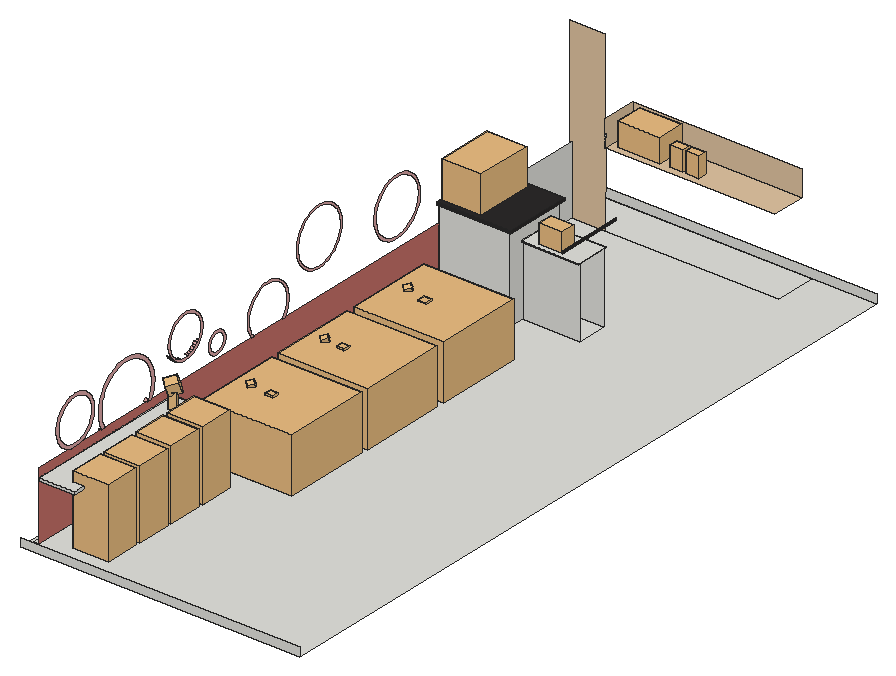
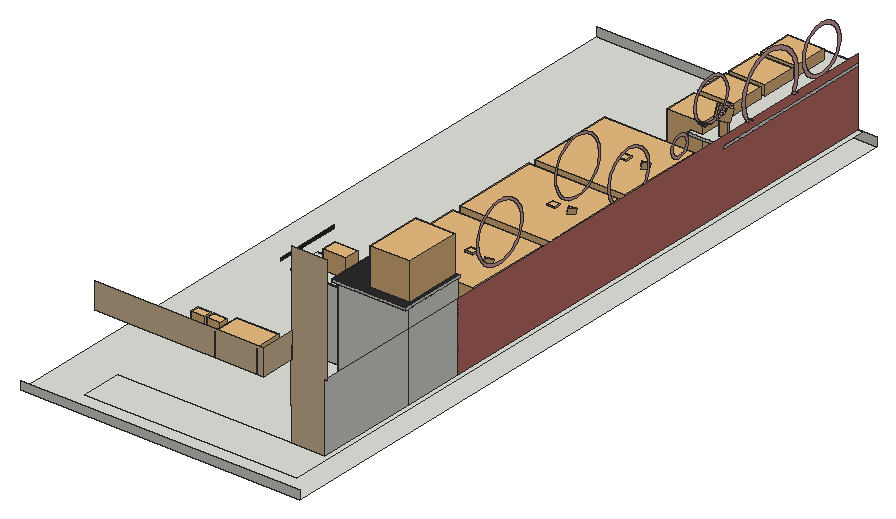
# SketchUp Ruby script. Lengths in inches.
U = 1.inch
M = Sketchup.active_model
def pt(a) = Geom::Point3d.new(a.map { |v| v * U })
def face(e, loops, mat)
  f = e.add_face(loops[0].map { |a| pt(a) })
  loops[1..].each { |l| e.add_face(l.map { |a| pt(a) }).erase! }
  f.material = f.back_material = mat if mat
  f
end
# faces: each face lists its corners as indices into pts; further lists are holes
def faces(e, pts, list, mat = nil) = list.each { |f| face(e, (f[0].is_a?(Array) ? f : [f]).map { |l| l.map { |i| pts[i] } }, mat) }
# xy, xz, yz: faces in a plane at the given z, y or x. An outline is a flat list of corners, or four numbers for a rectangle; further outlines are holes
def ring(l) = l.size == 4 ? [[l[0], l[1]], [l[2], l[1]], [l[2], l[3]], [l[0], l[3]]] : l.each_slice(2).to_a
def flat(e, list, mat, &to3) = list.each { |f| face(e, (f[0].is_a?(Array) ? f : [f]).map { |l| ring(l).map { |u, v| to3.(u, v) } }, mat) }
def xy(e, z, list, mat = nil) = flat(e, list, mat) { |x, y| [x, y, z] }
def xz(e, y, list, mat = nil) = flat(e, list, mat) { |x, z| [x, y, z] }
def yz(e, x, list, mat = nil) = flat(e, list, mat) { |y, z| [x, y, z] }
def lines(e, pts, list) = list.each { |a, b| e.add_line(pt(pts[a]), pt(pts[b])) }
# prism: a flat outline (further loops are holes) pulled along v
def prism(e, loops, v, mat = nil)
  f = face(e, loops, mat); d = Geom::Vector3d.new(v.map { |x| x * U })
  f.pushpull(f.normal.samedirection?(d) ? d.length : -d.length)
end
def box(e, o, s, mat = nil) = prism(e, [[o, [o[0] + s[0], o[1], o[2]], [o[0] + s[0], o[1] + s[1], o[2]], [o[0], o[1] + s[1], o[2]]]], [0, 0, s[2]], mat)
def at(x, y, z, deg = 0) = Geom::Transformation.translation(pt([x, y, z])) * Geom::Transformation.rotation(ORIGIN, Z_AXIS, deg.degrees)
def axes(o, x, y, z) = Geom::Transformation.new([*x, 0, *y, 0, *z, 0, *pt(o).to_a, 1])
def part(name) = M.definitions.add(name)
# library, detail: a bought-in or finely detailed component or shape, given as its bounding box
def library(name, o, s) = part(name).tap { |d| box(d.entities, o, s) }
def detail(e, o, s) = box(e.add_group.entities, o, s)
def put(e, d, t, mat = nil) = e.add_instance(d, t).tap { |i| i.material = mat if mat }
def group(e, t, mat = nil) = e.add_group.tap { |g| g.transformation = t; g.material = mat if mat }.entities
root = M.entities
M.materials.add("Generic").color = [224, 169, 169]
M.materials.add("Generic\#1").color = [44, 42, 42]
M.materials.add("Generic\#3").color = [224, 196, 161]
M.materials.add("Material__1").color = [51, 42, 44]
M.materials.add("Material__2").color = [97, 132, 37]
M.materials.add("[Wood Floor Dark]").color = [198, 114, 106]
c1 = library("\#1",[-138.85,-135.75,0],[277.7,270.97,9.64])
c2 = library("\#2",[-34.84,-73.35,-33.91],[69.68,146.26,68.31])
c3 = library("\#5",[-4127.85,-1300.75,-2324.72],[5349.84,4521.24,5423.31])
c4 = part("\#3")
put(c4.entities,c3,at(450.18,-1111.4375,0),"Material__2")
c5 = part("12")
put(c5.entities,c1,axes([-49.79,-36.9375,349.64],[0.59279,0,0],[0,0.59279,0],[0,0,0.59279]),"Material__1")
put(c5.entities,c2,axes([-39.24,-18.18,177.19],[1.20819,-2.09264,0],[0,0,2.41638],[2.09264,1.20819,0]))
put(c5.entities,c4,axes([-83.44,-46.04,442.44],[-0.03636,-0.03293,-0.01473],[-0.00083,-0.02391,0.05549],[0.02997,-0.02791,-0.01158]))
c6 = library("Group\#636",[0,0,0],[15.67,22.625,14.53])
c7 = library("Group\#669",[0,0,0],[8.6,8.6,4.41])
c8 = library("Group",[-8.82,-17.72,0],[17.64,35.44,18.29])
c9 = library("Tissue box",[0,0,0],[4.59,4,6.84])
c10 = library("Group\#25",[0,0,0],[61.25,59.29,37.22])
c11 = library("Group\#26",[0,0,0],[61.25,59.29,37.22])
c12 = library("Group\#23",[0,0,0],[61.25,59.29,37.22])
c13 = library("Espresso+machine+low+poly",[-3.8125,0,0],[25.21,40.375,21.95])
c14 = library("Group\#670",[0,0,0],[21.93,14.72,17.62])
c15 = library("Countertop blender",[-3.14,-3.14,0],[6.83,6.28,15])
xy(root,-6,[[0,0,190,490.125]])
xy(root,0,[[9,0.4375,12.375,0.4375,12.375,453.375,153.2,453.375,153.2,481.125,9,481.125],[60.5625,351.3,99.75,371.55]])
xy(root,38.39,[[12.375,0.4375,36.5,114.5]])
xy(root,40.64,[[12.375,0.4375,36.5,114.5]])
xy(root,46.5,[[12.375,27.54,12.625,34.125],[12.375,53.23,12.9375,56.0625],[12.375,91.96,12.9375,94.93]])
xy(root,47.6875,[[60.5625,350.05,99.75,351.3],[60.5625,351.3,99.75,371.55],[60.5625,371.55,99.75,372.8]])
xy(root,48.3125,[[60.5625,350.05,99.75,372.8]])
xy(root,50.68,[[35.21,453.375,150.42,476.6875]],"Generic\#3")
xy(root,58.4375,[[12.375,338.55,62.5625,340.55],[12.375,340.55,60.5625,382.3],[60.5625,340.55,62.5625,384.3],[12.375,382.3,60.5625,384.3]])
xy(root,60.3125,[[12.375,338.55,62.5625,384.3]],"Generic\#1")
xz(root,0,[[0,-6,190,0]])
xz(root,0.4375,[[12.375,38.39,36.5,40.64]])
xz(root,114.5,[[12.375,38.39,36.5,40.64]])
xz(root,338.55,[[12.375,58.4375,62.5625,60.3125]],"Generic\#1")
xz(root,340.55,[[12.375,0,60.5625,58.4375]])
xz(root,350.05,[[60.5625,47.6875,99.75,48.3125]])
xz(root,351.3,[[60.5625,0,99.75,47.6875]])
xz(root,371.55,[[60.5625,0,99.75,47.6875]])
xz(root,372.8,[[60.5625,47.6875,99.75,48.3125]])
xz(root,382.3,[[12.375,0,60.5625,58.4375]])
xz(root,384.3,[[12.375,58.4375,62.5625,60.3125]])
xz(root,453.375,[[34.92,50.68,35.21,50.68,34.93,68.36,34.92,68.36]])
xz(root,453.375,[[12.375,0,34.875,0,35.29,46.12,35.21,50.68,34.92,50.68,34.92,68.36,34.93,68.36,34.875,71.49,34.875,120,10.6875,120,10.6875,46.5,12.375,46.5]],"Generic\#3")
xz(root,476.6875,[[35.21,50.68,150.42,50.68,150.42,68.36,34.93,68.36]],"Generic\#3")
xz(root,490.125,[[0,-6,190,0]])
yz(root,12,[[[305.99,52.23,308.22,52.44,310.42,52.9,312.54,53.61,314.58,54.5625,316.49,55.74,318.25,57.12,319.85,58.7,321.26,60.44,322.45,62.34,323.43,64.36,324.17,66.48,324.66,68.67,324.89,70.9,324.875,73.14,324.6,75.37,324.08,77.55,323.31,79.66,322.3,81.66,321.07,83.54,319.64,85.27,318.02,86.82,316.23,88.17,314.3,89.31,312.25,90.23,310.11,90.91,307.91,91.33,305.68,91.51,303.43,91.43,301.22,91.09,299.05,90.5,296.97,89.67,294.99,88.61,293.15,87.33,291.47,85.85,289.96,84.18,288.66,82.36,287.57,80.39,286.71,78.32,286.1,76.16,285.73,73.95,285.625,71.71,285.77,69.47,286.17,67.26,286.82,65.12,287.71,63.06,288.83,61.11,290.16,59.31,291.69,57.67,293.4,56.21,295.26,54.96,297.25,53.93,299.35,53.13,301.52,52.58,303.74,52.28],[305.93,53.75,303.86,53.8,301.8125,54.07,299.81,54.58,297.87,55.32,296.03,56.27,294.32,57.43,292.74,58.77,291.33,60.28,290.1,61.95,289.07,63.74,288.25,65.64,287.65,67.62,287.28,69.66,287.15,71.72,287.25,73.79,287.58,75.83,288.15,77.82,288.94,79.73,289.95,81.54,291.15,83.23,292.54,84.76,294.09,86.13,295.79,87.3125,297.61,88.29,299.53,89.06,301.53,89.6,303.58,89.91,305.64,89.99,307.71,89.83,309.74,89.43,311.71,88.81,313.6,87.96,315.38,86.91,317.03,85.66,318.53,84.23,319.85,82.64,320.98,80.9,321.91,79.05,322.62,77.11,323.11,75.1,323.36,73.04,323.375,70.97,323.15,68.92,322.7,66.9,322.02,64.94,321.12,63.08,320.02,61.33,318.72,59.72,317.25,58.26,315.62,56.99,313.86,55.9,311.98,55.03,310.02,54.375,307.99,53.95]]],"Generic")
yz(root,12.1875,[[[239.61,63.57,241.81,63.77,243.97,64.23,246.06,64.93,248.0625,65.86,249.94,67.02,251.68,68.38,253.25,69.93,254.64,71.65,255.82,73.52,256.77,75.51,257.5,77.59,257.98,79.75,258.22,81.94,258.2,84.15,257.93,86.34,257.41,88.49,256.66,90.5625,255.67,92.54,254.46,94.39,253.05,96.08,251.45,97.61,249.69,98.95,247.79,100.07,245.78,100.97,243.67,101.64,241.5,102.06,239.3,102.23,237.09,102.15,234.91,101.82,232.78,101.24,230.73,100.42,228.78,99.38,226.97,98.12,225.3125,96.66,223.83,95.02,222.55,93.22,221.48,91.29,220.64,89.25,220.03,87.125,219.67,84.95,219.5625,82.74,219.71,80.54,220.1,78.37,220.74,76.25,221.61,74.22,222.71,72.3125,224.03,70.53,225.53,68.92,227.21,67.49,229.05,66.25,231.01,65.24,233.07,64.45,235.21,63.91,237.4,63.61],[239.5625,64.78,237.49,64.82,235.44,65.1,233.4375,65.61,231.5,66.35,229.66,67.3,227.95,68.45,226.37,69.8,224.96,71.3125,223.73,72.98,222.7,74.77,221.88,76.67,221.28,78.65,220.91,80.6875,220.78,82.75,220.88,84.82,221.22,86.86,221.78,88.85,222.57,90.76,223.58,92.57,224.78,94.26,226.17,95.79,227.72,97.16,229.42,98.34,231.24,99.32,233.16,100.09,235.16,100.63,237.21,100.94,239.28,101.02,241.34,100.86,243.37,100.46,245.34,99.84,247.23,98.99,249.01,97.9375,250.66,96.6875,252.16,95.26,253.48,93.66,254.61,91.93,255.54,90.08,256.25,88.14,256.74,86.13,256.99,84.07,257,82,256.78,79.95,256.33,77.93,255.65,75.97,254.75,74.11,253.65,72.36,252.35,70.75,250.88,69.29,249.25,68.01,247.49,66.93,245.61,66.06,243.65,65.4,241.62,64.98]]],"Generic")
yz(root,12.375,[[340.55,0,382.3,46.5],[382.3,0,453.375,46.5],[0.4375,38.39,114.5,40.64],[340.55,46.5,382.3,58.4375],[338.55,58.4375,384.3,60.3125]])
yz(root,12.375,[[181.21,46.5,182.81,46.5,181.875,47.65,180.875,49.23,180.06,50.9,179.45,52.66,179.04,54.48,178.84,56.33,178.85,58.19,179.07,60.04,179.5,61.85,180.14,63.6,180.97,65.27,181.98,66.83,183.17,68.27,184.52,69.56,186,70.69,187.6,71.64,189.3,72.4,191.07,72.97,192.9,73.33,194.75,73.48,196.62,73.41,198.46,73.14,200.26,72.65,201.99,71.97,203.63,71.09,205.16,70.03,206.5625,68.8,207.8125,67.42,208.9,65.91,209.81,64.28,210.52,62.5625,211.04,60.77,211.34,58.93,211.4375,57.07,211.32,55.22,210.99,53.38,210.46,51.6,209.72,49.89,208.8,48.27,207.7,46.77,207.45,46.5,209.04,46.5,209.84,47.59,210.84,49.33,211.63,51.17,212.21,53.09,212.56,55.07,212.6875,57.07,212.58,59.07,212.25,61.05,211.7,62.97,210.93,64.82,209.95,66.58,208.78,68.2,207.4375,69.69,205.93,71.01,204.28,72.15,202.51,73.1,200.65,73.84,198.71,74.36,196.73,74.65,194.73,74.72,192.73,74.5625,190.76,74.18,188.85,73.57,187.02,72.74,185.3,71.72,183.7,70.5,182.26,69.11,180.98,67.57,179.89,65.89,178.99,64.1,178.31,62.21,177.84,60.26,177.6,58.27,177.59,56.27,177.81,54.27,178.25,52.32,178.91,50.42,179.79,48.62,180.86,46.93],[[152.02,49.25,152.83,49.33,153.61,49.5,154.38,49.76,155.11,50.09,155.8,50.51,156.44,51,157.02,51.55,157.54,52.17,157.99,52.84,158.36,53.56,158.65,54.31,158.85,55.09,158.97,55.88,159,56.6875,158.94,57.49,158.79,58.28,158.56,59.06,158.24,59.8,157.85,60.5,157.375,61.15,156.84,61.75,156.23,62.28,155.58,62.75,154.87,63.14,154.13,63.45,153.35,63.67,152.5625,63.81,151.76,63.87,150.95,63.83,150.16,63.7,149.38,63.49,148.63,63.2,147.92,62.82,147.25,62.37,146.64,61.84,146.09,61.26,145.61,60.61,145.2,59.92,144.87,59.18,144.62,58.42,144.46,57.625,144.38,56.82,144.4,56.02,144.5,55.22,144.69,54.4375,144.97,53.68,145.32,52.96,145.76,52.28,146.26,51.65,146.84,51.09,147.47,50.59,148.15,50.16,148.875,49.81,149.63,49.54,150.42,49.36,151.22,49.26],[151.32,50.75,150.68,50.83,150.06,50.98,149.45,51.19,148.875,51.47,148.33,51.81,147.83,52.21,147.375,52.66,146.97,53.16,146.63,53.7,146.35,54.27,146.125,54.87,145.97,55.49,145.89,56.13,145.88,56.77,145.94,57.41,146.07,58.03,146.27,58.64,146.53,59.23,146.85,59.78,147.24,60.29,147.68,60.76,148.16,61.18,148.69,61.54,149.26,61.83,149.85,62.07,150.47,62.24,151.1,62.34,151.74,62.37,152.38,62.33,153.01,62.22,153.63,62.04,154.22,61.79,154.78,61.48,155.3,61.11,155.78,60.68,156.21,60.21,156.58,59.6875,156.9,59.13,157.15,58.54,157.34,57.93,157.45,57.3,157.5,56.66,157.48,56.02,157.38,55.39,157.22,54.77,156.99,54.17,156.7,53.6,156.34,53.07,155.93,52.58,155.47,52.14,154.96,51.75,154.41,51.42,153.83,51.15,153.22,50.95,152.59,50.8125,151.96,50.75]]],"Generic")
yz(root,12.375,[[0.4375,0,340.55,0,340.55,46.5,0.4375,46.5,0.4375,40.64,114.5,40.64,114.5,38.39,0.4375,38.39]],"[Wood Floor Dark]")
yz(root,12.625,[[[27.54,46.5,34.125,46.5,35.01,46.69,36.33,47.11,37.61,47.625,38.84,48.25,40.02,48.99,41.125,49.8125,42.16,50.73,43.11,51.73,43.98,52.8125,44.75,53.96,45.42,55.17,45.98,56.4375,46.43,57.74,46.78,59.08,47,60.45,47.12,61.83,47.11,63.21,46.99,64.59,46.75,65.95,46.39,67.29,45.93,68.59,45.35,69.85,44.67,71.05,43.89,72.19,43.02,73.27,42.06,74.26,41.01,75.17,39.9,75.99,38.72,76.71,37.48,77.32,36.19,77.83,34.87,78.23,33.51,78.52,32.14,78.6875,30.76,78.74,29.38,78.68,28.01,78.49,26.66,78.2,25.34,77.79,24.05,77.26,22.82,76.64,21.65,75.91,20.54,75.08,19.5,74.16,18.55,73.16,17.6875,72.08,16.92,70.93,16.25,69.72,15.68,68.45,15.23,67.15,14.89,65.81,14.66,64.44,14.55,63.06,14.55,61.68,14.68,60.3,14.92,58.94,15.27,57.6,15.74,56.3,16.3125,55.04,16.99,53.84,17.77,52.7,18.65,51.625,19.61,50.63,20.65,49.72,21.77,48.9,22.95,48.18,24.1875,47.57,25.47,47.06,26.8,46.66],[30.9,48.2,29.6875,48.24,28.49,48.39,27.3,48.64,26.14,48.99,25.02,49.43,23.9375,49.97,22.9,50.6,21.93,51.32,21.02,52.11,20.18,52.98,19.41,53.92,18.73,54.92,18.14,55.97,17.63,57.07,17.23,58.21,16.92,59.38,16.71,60.57,16.6,61.78,16.59,62.99,16.6875,64.19,16.89,65.39,17.1875,66.56,17.59,67.7,18.08,68.8,18.66,69.86,19.34,70.87,20.09,71.8125,20.93,72.69,21.83,73.49,22.8,74.22,23.83,74.86,24.9,75.4,26.03,75.86,27.18,76.22,28.36,76.48,29.56,76.64,30.77,76.7,31.98,76.65,33.18,76.5,34.36,76.25,35.52,75.9,36.64,75.46,37.73,74.92,38.76,74.29,39.73,73.57,40.65,72.78,41.49,71.91,42.25,70.97,42.93,69.97,43.53,68.92,44.03,67.82,44.4375,66.68,44.75,65.51,44.96,64.32,45.07,63.11,45.07,61.9,44.97,60.7,44.78,59.51,44.48,58.33,44.08,57.19,43.58,56.09,43,55.03,42.33,54.02,41.57,53.08,40.74,52.2,39.83,51.4,38.86,50.67,37.84,50.04,36.76,49.49,35.64,49.03,34.48,48.67,33.3,48.41,32.1,48.25]]],"Generic")
yz(root,12.9375,[[53.23,46.5,56.0625,46.5,55.2,47.85,54.5,49.29,53.91,50.78,53.4375,52.31,53.08,53.87,52.84,55.45,52.72,57.05,52.71,58.65,52.83,60.25,53.07,61.83,53.42,63.39,53.89,64.92,54.48,66.42,55.17,67.86,55.97,69.25,56.87,70.57,57.87,71.82,58.96,73,60.13,74.09,61.39,75.08,62.71,75.99,64.1,76.79,65.54,77.48,67.03,78.0625,68.5625,78.53,70.125,78.89,71.71,79.125,73.31,79.24,74.91,79.24,76.51,79.12,78.09,78.875,79.65,78.52,81.18,78.04,82.67,77.45,84.11,76.75,85.5,75.95,86.82,75.04,88.07,74.04,89.24,72.95,90.32,71.77,91.32,70.51,92.21,69.1875,93.01,67.8,93.7,66.35,94.28,64.86,94.74,63.33,95.09,61.76,95.32,60.18,95.4375,58.58,95.43,56.98,95.3,55.38,95.06,53.8,94.69,52.24,94.21,50.71,93.62,49.23,92.92,47.79,91.96,46.5,94.93,46.5,94.96,46.54,95.8,48.26,96.46,49.91,96.99,51.61,97.4,53.35,97.67,55.1,97.8125,56.88,97.82,58.66,97.7,60.4375,97.44,62.2,97.05,63.93,96.53,65.64,95.89,67.3,95.125,68.91,94.24,70.45,93.24,71.92,92.14,73.32,90.93,74.63,89.63,75.84,88.24,76.96,86.77,77.97,85.23,78.86,83.63,79.64,81.97,80.29,80.27,80.82,78.54,81.22,76.78,81.49,75,81.625,73.22,81.63,71.45,81.5,69.69,81.23,67.95,80.84,66.25,80.32,64.59,79.67,62.98,78.9,61.44,78.01,59.97,77,58.58,75.89,57.27,74.68,56.0625,73.38,54.95,71.99,53.95,70.52,53.06,68.97,52.29,67.37,51.64,65.71,51.12,64.01,50.72,62.27,50.46,60.51,50.33,58.74,50.33,56.96,50.47,55.18,50.73,53.42,51.13,51.69,51.66,49.99,52.32,48.33,53.12,46.68],[[123.83,58.04,125.5,58.09,127.15,58.33,128.76,58.76,130.32,59.36,131.8,60.15,133.17,61.09,134.4375,62.1875,135.5625,63.42,136.54,64.77,137.36,66.23,138.01,67.77,138.48,69.375,138.76,71.02,138.85,72.69,138.75,74.36,138.47,76,137.99,77.61,137.34,79.14,136.52,80.6,135.53,81.95,134.4,83.18,133.14,84.27,131.75,85.21,130.28,85.99,128.72,86.59,127.1,87.01,125.45,87.25,123.78,87.29,122.11,87.15,120.48,86.8125,118.89,86.29,117.37,85.6,115.94,84.73,114.62,83.71,113.42,82.54,112.37,81.25,111.47,79.84,110.73,78.34,110.17,76.76,109.8,75.14,109.61,73.48,109.61,71.81,109.8,70.15,110.1875,68.52,110.75,66.95,111.49,65.45,112.4,64.04,113.46,62.75,114.66,61.59,115.98,60.57,117.41,59.71,118.93,59.02,120.52,58.51,122.16,58.18],[123.87,59.48,122.36,59.61,120.89,59.91,119.46,60.37,118.09,60.99,116.79,61.77,115.6,62.68,114.52,63.73,113.5625,64.9,112.75,66.16,112.08,67.51,111.57,68.93,111.23,70.39,111.05,71.89,111.05,73.4,111.22,74.89,111.56,76.36,112.0625,77.78,112.73,79.13,113.54,80.4,114.49,81.57,115.57,82.62,116.76,83.54,118.05,84.32,119.41,84.95,120.85,85.41,122.32,85.72,123.82,85.85,125.33,85.81,126.82,85.59,128.27,85.21,129.68,84.67,131.01,83.97,132.25,83.12,133.39,82.14,134.41,81.03,135.3,79.8125,136.04,78.5,136.63,77.12,137.06,75.67,137.32,74.19,137.41,72.6875,137.32,71.18,137.07,69.7,136.65,68.25,136.0625,66.87,135.33,65.55,134.44,64.33,133.43,63.22,132.29,62.24,131.05,61.38,129.72,60.68,128.32,60.13,126.86,59.74,125.37,59.53]]],"Generic")
yz(root,36.5,[[0.4375,38.39,114.5,40.64]])
yz(root,60.5625,[[340.55,0,351.3,0,351.3,47.6875,350.05,47.6875,350.05,48.3125,372.8,48.3125,372.8,47.6875,371.55,47.6875,371.55,0,382.3,0,382.3,58.4375,340.55,58.4375],[350.05,47.6875,372.8,48.3125]])
yz(root,62.5625,[[338.55,58.4375,384.3,60.3125]],"Generic\#1")
yz(root,97.8125,[[338.55,58.4375,384.3,60.3125]],"Generic\#1")
p = [[10.6875,53.12,46.68],[10.6875,53.23,46.5],[12.375,53.23,46.5],[12.9375,53.23,46.5],[12.9375,53.12,46.68],[10.6875,56.0625,46.5],
  [10.6875,55.2,47.85],[12.9375,55.2,47.85],[12.9375,56.0625,46.5],[12.375,56.0625,46.5],[10.6875,92.92,47.79],[10.6875,91.96,46.5],
  [12.375,91.96,46.5],[12.9375,91.96,46.5],[12.9375,92.92,47.79],[10.6875,94.93,46.5],[10.6875,94.96,46.54],[12.9375,94.96,46.54],
  [12.9375,94.93,46.5],[12.375,94.93,46.5],[34.93,453.375,68.36],[35.21,453.375,50.68],[35.21,476.6875,50.68],[34.93,476.6875,68.36],
  [10.6875,128.32,60.13],[10.6875,126.86,59.74],[12.9375,126.86,59.74],[12.9375,128.32,60.13],[10.6875,120.89,59.91],[10.6875,119.46,60.37],
  [12.9375,119.46,60.37],[12.9375,120.89,59.91],[10.6875,129.72,60.68],[12.9375,129.72,60.68],[10.6875,131.8,60.15],[10.6875,133.17,61.09],
  [12.9375,133.17,61.09],[12.9375,131.8,60.15],[10.6875,118.09,60.99],[12.9375,118.09,60.99],[10.6875,114.66,61.59],[10.6875,115.98,60.57],
  [12.9375,115.98,60.57],[12.9375,114.66,61.59],[10.6875,131.05,61.38],[12.9375,131.05,61.38],[10.6875,116.79,61.77],[12.9375,116.79,61.77],
  [10.6875,134.4375,62.1875],[12.9375,134.4375,62.1875],[10.6875,132.29,62.24],[12.9375,132.29,62.24],[10.6875,113.46,62.75],[12.9375,113.46,62.75],
  [10.6875,115.6,62.68],[12.9375,115.6,62.68],[10.6875,133.43,63.22],[12.9375,133.43,63.22],[10.6875,135.5625,63.42],[12.9375,135.5625,63.42],
  [10.6875,114.52,63.73],[12.9375,114.52,63.73],[10.6875,112.4,64.04],[12.9375,112.4,64.04],[10.6875,134.44,64.33],[12.9375,134.44,64.33],
  [10.6875,136.54,64.77],[12.9375,136.54,64.77],[10.6875,113.5625,64.9],[12.9375,113.5625,64.9],[10.6875,111.49,65.45],[12.9375,111.49,65.45],
  [83.22,347.8,17.61],[83.29,347.8,17.61],[83.29,347.87,17.61]]
faces(root,p,[[0,1,2,3,4],[5,6,7,8,9],[10,11,12,13,14],[15,16,17,18,19],[24,25,26,27],[28,29,30,31],[32,24,27,33],[34,35,36,37],
  [29,38,39,30],[40,41,42,43],[44,32,33,45],[38,46,47,39],[35,48,49,36],[50,44,45,51],[52,40,43,53],[46,54,55,47],
  [56,50,51,57],[48,58,59,49],[54,60,61,55],[62,52,53,63],[64,56,57,65],[58,66,67,59],[60,68,69,61],[70,62,63,71]],"Generic")
faces(root,p,[[20,21,22,23]],"Generic\#3")
lines(root,p,[[72,73],[73,74],[74,72]])
put(root,c5,axes([21,105.35,40.64],[0.02931,0,0],[0,0.02931,0],[0,0,0.02931]))
put(root,c6,axes([13.875,340.96,61.0625],[1.7056,0,0],[0,1.7056,0],[0,0,1.7056]))
put(root,c5,axes([34.65,287.27,30.35],[0.01602,0,0],[0,0.01602,0],[0,0,0.01602]))
put(root,c5,axes([34.65,216.64,30.35],[0.01602,0,0],[0,0.01602,0],[0,0,0.01602]))
put(root,c5,axes([34.65,154.08,30.35],[0.01602,0,0],[0,0.01602,0],[0,0,0.01602]))
put(root,c7,at(36.44,274.42,30))
put(root,c8,axes([53.17,100.1,23.5625],[0,-1.33,0],[0,0,1.33],[-1.33,0,0]))
put(root,c8,axes([53.17,73.47,23.5625],[0,-1.33,0],[0,0,1.33],[-1.33,0,0]))
put(root,c8,axes([53.17,46.85,23.5625],[0,-1.33,0],[0,0,1.33],[-1.33,0,0]))
put(root,c8,axes([53.17,20.22,23.5625],[0,-1.33,0],[0,0,1.33],[-1.33,0,0]))
put(root,c9,axes([43.7,214.08,30],[1.16688,0,0],[0,1.16688,0],[0,0,1.16688]))
put(root,c9,axes([46,150.37,30],[1.16688,0,0],[0,1.16688,0],[0,0,1.16688]))
put(root,c9,axes([46.125,280.59,30],[1.16688,0,0],[0,1.16688,0],[0,0,1.16688]))
put(root,c10,at(23.33,254.22,0))
put(root,c11,at(23.33,189.41,0))
put(root,c12,at(23.33,125.28,0))
put(root,c13,axes([68.62,460.83,50.68],[0,0.73,0],[-0.71159,0,0],[0,0,0.73]),"Generic\#3")
put(root,c14,axes([69.9,353.02,48.3125],[0.72,0,0],[0,0.72,0],[0,0,0.72]))
put(root,c15,axes([79.07,461.25,50.68],[1.32741,0,0],[0,0.903,0],[0,0,0.903]))
put(root,c15,axes([89.69,461.25,50.68],[1.32741,0,0],[0,0.903,0],[0,0,0.903]))
